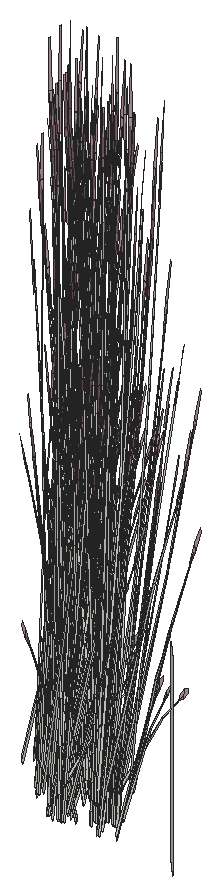
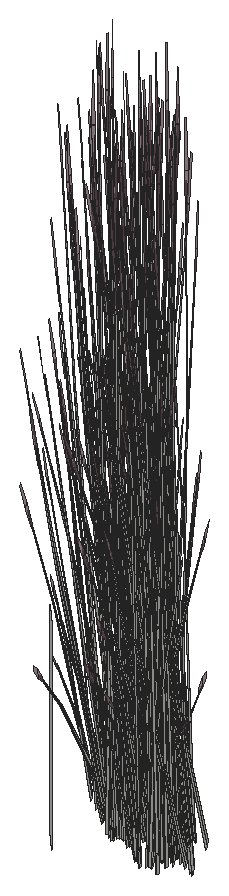
# SketchUp Ruby script. Lengths in inches.
U = 1.inch
M = Sketchup.active_model
def pt(a) = Geom::Point3d.new(a.map { |v| v * U })
def face(e, loops, mat)
  f = e.add_face(loops[0].map { |a| pt(a) })
  loops[1..].each { |l| e.add_face(l.map { |a| pt(a) }).erase! }
  f.material = f.back_material = mat if mat
  f
end
# faces: each face lists its corners as indices into pts; further lists are holes
def faces(e, pts, list, mat = nil) = list.each { |f| face(e, (f[0].is_a?(Array) ? f : [f]).map { |l| l.map { |i| pts[i] } }, mat) }
# xy, xz, yz: faces in a plane at the given z, y or x. An outline is a flat list of corners, or four numbers for a rectangle; further outlines are holes
def ring(l) = l.size == 4 ? [[l[0], l[1]], [l[2], l[1]], [l[2], l[3]], [l[0], l[3]]] : l.each_slice(2).to_a
def flat(e, list, mat, &to3) = list.each { |f| face(e, (f[0].is_a?(Array) ? f : [f]).map { |l| ring(l).map { |u, v| to3.(u, v) } }, mat) }
def xy(e, z, list, mat = nil) = flat(e, list, mat) { |x, y| [x, y, z] }
def xz(e, y, list, mat = nil) = flat(e, list, mat) { |x, z| [x, y, z] }
def yz(e, x, list, mat = nil) = flat(e, list, mat) { |y, z| [x, y, z] }
def lines(e, pts, list) = list.each { |a, b| e.add_line(pt(pts[a]), pt(pts[b])) }
# prism: a flat outline (further loops are holes) pulled along v
def prism(e, loops, v, mat = nil)
  f = face(e, loops, mat); d = Geom::Vector3d.new(v.map { |x| x * U })
  f.pushpull(f.normal.samedirection?(d) ? d.length : -d.length)
end
def box(e, o, s, mat = nil) = prism(e, [[o, [o[0] + s[0], o[1], o[2]], [o[0] + s[0], o[1] + s[1], o[2]], [o[0], o[1] + s[1], o[2]]]], [0, 0, s[2]], mat)
def at(x, y, z, deg = 0) = Geom::Transformation.translation(pt([x, y, z])) * Geom::Transformation.rotation(ORIGIN, Z_AXIS, deg.degrees)
def axes(o, x, y, z) = Geom::Transformation.new([*x, 0, *y, 0, *z, 0, *pt(o).to_a, 1])
def part(name) = M.definitions.add(name)
# library, detail: a bought-in or finely detailed component or shape, given as its bounding box
def library(name, o, s) = part(name).tap { |d| box(d.entities, o, s) }
def detail(e, o, s) = box(e.add_group.entities, o, s)
def put(e, d, t, mat = nil) = e.add_instance(d, t).tap { |i| i.material = mat if mat }
def group(e, t, mat = nil) = e.add_group.tap { |g| g.transformation = t; g.material = mat if mat }.entities
root = M.entities
M.materials.add("LightPink_Translucent").color = [144, 107, 117]
M.materials["LightPink_Translucent"].alpha = 0.75
c1 = part("blade")
p = [[2.15,0.21,22],[0,0.17,0],[0.09,0.45,0],[2.18,0.31,22],[2.29,0.31,22],[0.38,0.45,0],
  [2.48,0.24,33],[2.49,0.24,33],[2.48,0.22,33]]
faces(c1.entities,p,[[0,1,2,3],[4,5,2,3],[6,3,4,7],[8,0,3,6]])
c2 = part("seeds")
p = [[0.3,-0.1,1.38],[-0.01,-0.03,1.59],[-0.01,-0.03,0.03],[0.14,-0.07,-0.07],[0.29,-0.03,3],[0.15,0.01,3.11]]
faces(c2.entities,p,[[0,1,2,3],[1,0,4,5]],"LightPink_Translucent")
c3 = part("blade with seeds")
put(c3.entities,c1,at(0,0,0))
put(c3.entities,c2,axes([2.4,0.25,30.99],[1.5799,-0.05474,1.17369],[-0.12525,1.92788,0.29478],[-0.07173,-0.02425,1.56792]))
p = [[369.42,355.39,618],[371.24,353.33,618],[371.24,353.33,636],[369.42,355.39,636]]
faces(root,p,[[0,1,2,3]])
put(root,c3,axes([359.65,352.5625,623.05],[0.23881,-0.24554,0.35414],[0.22606,0.28036,-0.4572],[-0.0344,0.14245,0.87481]))
put(root,c3,axes([357.41,354.85,622.73],[0.12963,0.31798,0.0643],[-0.23638,0.15564,0.50621],[0.1042,-0.03071,0.77189]))
put(root,c3,axes([361.25,351.21,620.84],[-0.00964,-0.43909,1.41272],[0.43635,0.11382,0.59816],[-0.1032,0.24027,1.3335]))
put(root,c3,axes([356.86,355.74,623.03],[0.0189,-0.47427,-0.1216],[0.35781,0.01296,-0.67495],[0.13781,0.03295,1.02557]))
put(root,c3,axes([357.26,354.86,623.03],[-0.17758,-0.42229,-0.1216],[0.31518,-0.20752,-0.67495],[0.13282,-0.05572,1.02557]))
put(root,c3,axes([362.3,353.98,620.59],[0.12266,0.03828,1.43002],[0.07906,0.39104,-0.30754],[-0.16661,0.0732,0.61141]))
put(root,c3,axes([357.38,354.74,622.73],[-0.09971,0.42522,0.48003],[-0.32782,-0.1454,0.3958],[0.12892,-0.02555,0.9933]))
put(root,c3,axes([359,355.04,620.38],[-0.44609,-0.09826,0.49198],[0.09078,-0.55493,0.19306],[0.06519,0.05359,1.70813]))
put(root,c3,axes([359.61,356.53,620.47],[0.37926,-0.12378,0.17642],[0.09365,0.46065,0.35086],[-0.03382,-0.06712,1.60407]))
put(root,c3,axes([359.5,352.63,623.4],[0.3879,0.02311,-0.13498],[-0.0106,0.43749,-0.74919],[-0.02694,0.1685,1.13838]))
put(root,c3,axes([363.39,352.72,621.34],[0.10032,-0.06746,1.77064],[0.0346,0.47103,0.13857],[-0.2173,0.0625,0.63284]))
put(root,c3,axes([361.01,351.77,620.67],[0.04113,0.53214,-0.29095],[-0.42835,0.03218,-0.50002],[-0.07543,0.07088,1.59708]))
put(root,c3,axes([359.125,355.28,620.21],[0.39487,0,0],[0,0.48281,0],[0,0,1.78407]))
put(root,c3,axes([358.74,354.75,620.72],[-0.21202,-0.39143,0.44739],[0.32115,-0.27564,-0.21531],[0.06861,0.04843,1.43643]))
put(root,c3,axes([358.36,354.84,620.67],[-0.04113,-0.53214,-0.29095],[0.42835,-0.03218,-0.50002],[0.07543,-0.07088,1.59708]))
put(root,c3,axes([360.74,356.55,620.47],[0.10196,-0.46348,0.17642],[0.3731,0.13116,0.35086],[-0.06445,0.00226,1.60407]))
put(root,c3,axes([362.31,353.04,622.72],[-0.05763,0.06055,1.74944],[0.0049,0.44239,-0.27667],[-0.13211,0.05753,0.14031]))
put(root,c3,axes([357.25,354.5,622.68],[0.09562,-0.42421,-0.51099],[0.32782,0.1454,-0.3958],[0.13199,-0.0389,0.97773]))
put(root,c3,axes([360.47,355.59,620.3],[-0.32829,-0.4014,-0.06131],[0.32849,-0.40164,0],[-0.01146,-0.01402,1.75571]))
put(root,c3,axes([358.07,354.77,620.77],[-0.21807,0.07699,1.1486],[0.10265,-0.31819,0.84392],[0.11568,0.02177,0.25299]))
put(root,c3,axes([362.49,352.79,622.53],[-0.29332,-0.1301,-0.35414],[0.08555,-0.37955,0.4572],[-0.11809,0.0348,0.87481]))
put(root,c3,axes([358.3,353.67,620.03],[0.32928,0.11539,-0.30978],[-0.08291,0.40636,0.30978],[0.06638,-0.04686,1.38974]))
put(root,c3,axes([357.45,354.69,622.53],[0.29332,0.1301,-0.35414],[-0.08555,0.37955,0.4572],[0.11809,-0.0348,0.87481]))
put(root,c3,axes([359.81,355.13,620.36],[0.15345,0.52148,0.45755],[-0.43845,0.18134,0.17955],[0.00536,-0.09582,1.58856]))
put(root,c3,axes([359.74,355.07,620.21],[0.17124,-0.42022,-0.44739],[0.35581,0.20224,0.21531],[0,-0.09687,1.43643]))
put(root,c3,axes([360.18,356.42,620.2],[-0.11516,-0.40207,0],[0.32884,-0.1408,0],[0,0,1.54371]))
put(root,c3,axes([361.67,353.49,622.71],[0.04504,0.01251,1.77383],[0.13934,0.41205,-0.16761],[-0.0922,0.10815,0.31391]))
put(root,c3,axes([362.7,352.98,622.68],[-0.09562,0.42421,-0.51099],[-0.32782,-0.1454,-0.3958],[-0.13199,0.0389,0.97773]))
put(root,c3,axes([357.6,354.62,619.98],[-0.22732,0.05597,1.41583],[-0.03618,-0.44548,0.08104],[0.15921,-0.06743,0.80566]))
put(root,c3,axes([358.89,354.64,620.62],[0.06809,-0.4162,0.1448],[0.33266,0.07225,-0.41347],[0.06054,0.04274,1.26744]))
put(root,c3,axes([361.44,353.06,620.375],[0.22066,0.46731,0],[-0.36918,0.26061,-0.51607],[-0.08408,0.05936,1.63711]))
put(root,c3,axes([357.85,354.33,619.49],[-0.01845,-0.0708,1.76342],[0.12793,-0.41416,-0.26939],[0.12905,-0.00596,0.30037]))
put(root,c3,axes([362.53,352.95,619.49],[0.00895,0.0735,1.76342],[-0.18044,0.38382,-0.26939],[-0.12817,-0.01935,0.30037]))
put(root,c3,axes([357.97,356.11,622.71],[-0.03191,-0.04083,1.77383],[0.06981,-0.43764,-0.16761],[0.12571,-0.02796,0.31391]))
put(root,c3,axes([360.32,353.26,623.0625],[-0.34777,-0.12192,0.53283],[0.11892,-0.40083,0.43934],[0.0209,0.15763,1.10256]))
put(root,c3,axes([356.65,354.22,621.875],[-0.14639,0.01056,1.71376],[0.09712,-0.45778,0.13857],[0.20862,0.02831,0.73262]))
put(root,c3,axes([360.22,353.29,622.73],[-0.26007,0.1585,0.0643],[-0.12729,-0.28902,0.50621],[0.02512,0.1274,0.77189]))
put(root,c3,axes([359.36,353.92,620.48],[-0.33032,-0.23318,0.49651],[0.19744,-0.41812,0],[0.07523,0.05311,1.57504]))
put(root,c3,axes([361.09,351.87,620.62],[0.26075,0.2802,0.1448],[-0.2175,0.31612,-0.41347],[-0.06054,0.04274,1.26744]))
put(root,c3,axes([362.05,354.79,620.77],[0.14709,-0.21136,1.1486],[0.05804,0.3346,0.84392],[-0.1063,0.05991,0.25299]))
put(root,c3,axes([359.07,356.35,620.18],[0.37054,-0.15823,-0.19198],[0.1302,0.45581,0.00008],[0.0409,-0.01749,1.73897]))
put(root,c3,axes([357.19,354.65,622.98],[0.31014,-0.20596,-0.71045],[0.17284,0.42397,0.08574],[0.14985,-0.04816,1.00501]))
put(root,c3,axes([360.36,355.18,620.21],[0,-0.53961,0],[0.44133,0,0],[0,0,1.79456]))
put(root,c3,axes([361.17,352.76,620.33],[0.44186,0.15158,0.30756],[-0.11054,0.54181,-0.36492],[-0.07313,0.06781,1.64885]))
put(root,c3,axes([362.68,352.62,623.03],[0.17758,0.42229,-0.1216],[-0.31518,0.20752,-0.67495],[-0.13282,0.05572,1.02557]))
put(root,c3,axes([359.95,355.27,620.43],[0.39767,0.22603,0.24065],[-0.19139,0.46966,0.50002],[0,-0.10827,1.60543]))
put(root,c3,axes([359.82,354.96,620.72],[-0.38326,0.02879,0.44739],[-0.03466,-0.47788,-0.21531],[0.06861,-0.04843,1.43643]))
put(root,c3,axes([362.54,352.625,622.73],[-0.12963,-0.31798,0.0643],[0.23638,-0.15564,0.50621],[-0.1042,0.03071,0.77189]))
put(root,c3,axes([361.36,352.73,620.48],[0.33032,-0.23318,0.49651],[0.19744,0.41812,0],[-0.07523,0.05311,1.57504]))
put(root,c3,axes([362.6,353.88,622.53],[-0.30722,0.06665,-0.35414],[-0.08112,-0.381,0.4572],[-0.08804,0.10234,0.87481]))
put(root,c3,axes([359.64,354.14,620.47],[-0.10196,0.46348,0.17642],[-0.3731,-0.13116,0.35086],[0.06445,-0.00226,1.60407]))
put(root,c3,axes([357.66,355.28,620.59],[-0.085,-0.1147,1.43002],[0.1106,-0.37943,-0.30754],[0.17198,0.0514,0.61141]))
put(root,c3,axes([362.64,353.8,622.73],[-0.08753,-0.42921,0.48003],[0.34336,-0.07449,0.3958],[-0.1012,0.10094,0.9933]))
put(root,c3,axes([360.77,354.16,620.47],[-0.37926,0.12378,0.17642],[-0.09365,-0.46065,0.35086],[0.03382,0.06712,1.60407]))
put(root,c3,axes([361.16,351.56,620.21],[-0.17124,0.42022,-0.44739],[-0.35581,-0.20224,0.21531],[0,0.09687,1.43643]))
put(root,c3,axes([362.57,353.72,622.73],[-0.2423,-0.19613,0.0643],[0.14107,-0.2793,0.50621],[-0.07768,0.0903,0.77189]))
put(root,c3,axes([359.66,354.13,620.03],[0.08291,0.40636,-0.30978],[-0.32928,0.11539,0.30978],[0.06638,0.04686,1.38974]))
put(root,c3,axes([360.15,354.84,620.36],[-0.29264,0.42323,0.45755],[-0.34767,-0.3736,0.17955],[0.07055,-0.04224,1.58856]))
put(root,c3,axes([358.85,354.78,620.67],[0.35635,-0.30962,-0.29095],[0.23697,0.43749,-0.50002],[0.08792,0.04443,1.59708]))
put(root,c3,axes([359.91,354.72,623.05],[-0.30722,0.06665,0.35414],[-0.08112,-0.381,-0.4572],[0.08804,-0.10234,0.87481]))
put(root,c3,axes([360.32,352.96,623.05],[0.1064,-0.35863,0.35414],[0.31043,0.1046,-0.4572],[0.02846,0.14439,0.87481]))
put(root,c3,axes([362.8,352.74,623.05],[0.29332,0.1301,0.35414],[-0.08555,0.37955,-0.4572],[-0.11809,0.0348,0.87481]))
put(root,c3,axes([360.53,355.05,620.38],[-0.44609,-0.09826,0.49198],[0.09078,-0.55493,0.19306],[0.06519,0.05359,1.70813]))
put(root,c3,axes([360.89,352.37,620.29],[0.15345,0.53576,-0.06012],[-0.43845,0.18773,0],[0.00536,0.01871,1.72173]))
put(root,c3,axes([360.66,355.3,620.21],[0.39487,0,0],[0,0.48281,0],[0,0,1.78407]))
put(root,c3,axes([362.16,351.66,620.2],[-0.44111,-0.00373,-0.04976],[0,-0.52122,0.49943],[-0.01386,0.11865,1.58352]))
put(root,c3,axes([360.28,354.76,620.72],[-0.21202,-0.39143,0.44739],[0.32115,-0.27564,-0.21531],[0.06861,0.04843,1.43643]))
put(root,c3,axes([359.89,354.86,620.67],[-0.04113,-0.53214,-0.29095],[0.42835,-0.03218,-0.50002],[0.07543,-0.07088,1.59708]))
put(root,c3,axes([357.95,354.5,619.59],[-0.3474,0.18671,1.28929],[-0.11057,-0.53572,0.50096],[0.21332,0.00891,1.46642]))
put(root,c3,axes([360.74,354.24,623.65],[0.2439,-0.26754,-0.06488],[0.22348,0.29302,-0.29416],[0.01573,0.08303,0.97024]))
put(root,c3,axes([363.23,354.51,620.02],[-0.33032,-0.23318,-0.49651],[0.19744,-0.41812,0],[-0.07523,-0.05311,1.57504]))
put(root,c3,axes([359.55,353.67,620.375],[0.22066,-0.46731,0],[0.36918,0.26061,-0.51607],[0.08408,0.05936,1.63711]))
put(root,c3,axes([359.84,353.68,620.03],[0.32928,0.11539,-0.30978],[-0.08291,0.40636,0.30978],[0.06638,-0.04686,1.38974]))
put(root,c3,axes([361.02,352.54,620.2],[0.35581,0.20937,0],[-0.17124,0.43505,0],[0,0,1.74954]))
put(root,c3,axes([363.43,354.79,620.375],[-0.22066,0.46731,0],[-0.36918,-0.26061,-0.51607],[-0.08408,-0.05936,1.63711]))
put(root,c3,axes([359.75,353.95,620.02],[0.33032,0.23318,-0.49651],[-0.19744,0.41812,0],[0.07523,0.05311,1.57504]))
put(root,c3,axes([360.22,353.12,623.03],[0.34538,-0.21713,-0.1216],[0.16972,0.38536,-0.67495],[0.04557,0.16239,1.02557]))
put(root,c3,axes([362.07,351.74,620.03],[-0.24637,0.29097,-0.30978],[-0.24637,-0.29097,0.30978],[0,0.09372,1.38974]))
put(root,c3,axes([360.42,354.65,620.62],[0.06809,-0.4162,0.1448],[0.33266,0.07225,-0.41347],[0.06054,0.04274,1.26744]))
put(root,c3,axes([359.96,355.63,623.05],[-0.29332,-0.1301,0.35414],[0.08555,-0.37955,-0.4572],[0.11809,-0.0348,0.87481]))
put(root,c3,axes([362.85,353.65,623.05],[0.30722,-0.06665,0.35414],[0.08112,0.381,-0.4572],[-0.08804,0.10234,0.87481]))
put(root,c3,axes([361.36,351.6875,620.09],[0.12941,0.42699,-0.69212],[-0.37279,0.15378,-0.18165],[0.0143,0.14459,1.52773]))
put(root,c3,axes([360.83,355.125,620.26],[-0.21881,-0.29821,-0.06488],[0.23965,-0.27324,-0.29416],[0.0679,-0.01924,0.97024]))
put(root,c3,axes([360.9,353.93,620.48],[-0.33032,-0.23318,0.49651],[0.19744,-0.41812,0],[0.07523,0.05311,1.57504]))
put(root,c3,axes([360.61,356.36,620.18],[0.37054,-0.15823,-0.19198],[0.1302,0.45581,0.00008],[0.0409,-0.01749,1.73897]))
put(root,c3,axes([360.1875,354.66,622.73],[0.2423,0.19613,0.0643],[-0.14107,0.2793,0.50621],[0.07768,-0.0903,0.77189]))
put(root,c3,axes([361.21,351.21,620.67],[0.39748,0.22252,-0.29095],[-0.19139,0.46966,-0.50002],[0.01249,0.11531,1.59708]))
put(root,c3,axes([364.13,353.6875,620.67],[-0.35635,0.30962,-0.29095],[-0.23697,-0.43749,-0.50002],[-0.08792,-0.04443,1.59708]))
put(root,c3,axes([360.12,354.58,622.73],[0.08753,0.42921,0.48003],[-0.34336,0.07449,0.3958],[0.1012,-0.10094,0.9933]))
put(root,c3,axes([363.32,354.34,620.03],[-0.08291,-0.40636,-0.30978],[0.32928,-0.11539,0.30978],[-0.06638,-0.04686,1.38974]))
put(root,c3,axes([362.24,351.75,620.02],[0,0.46636,-0.49651],[-0.39487,0,0],[0,0.10622,1.57504]))
put(root,c3,axes([361.18,353.16,622.73],[-0.35104,0.10702,0.48003],[-0.06092,-0.41983,0.3958],[0.08256,0.12373,0.9933]))
put(root,c3,axes([361.12,353.25,622.73],[-0.16041,0.29625,0.0643],[-0.22843,-0.17248,0.50621],[0.07385,0.09498,0.77189]))
put(root,c3,axes([360.23,355.75,622.73],[0.12963,0.31798,0.0643],[-0.23638,0.15564,0.50621],[0.1042,-0.03071,0.77189]))
put(root,c3,axes([360.08,355.76,623.03],[-0.17758,-0.42229,-0.1216],[0.31518,-0.20752,-0.67495],[0.13282,-0.05572,1.02557]))
put(root,c3,axes([360.2,355.64,622.73],[-0.09971,0.42522,0.48003],[-0.32782,-0.1454,0.3958],[0.12892,-0.02555,0.9933]))
put(root,c3,axes([364.53,353.83,620.46],[-0.34464,-0.37536,-0.25192],[0.29,-0.42149,0.5513],[-0.0928,0.04391,1.68216]))
put(root,c3,axes([361.19,354.14,620.03],[0.08291,0.40636,-0.30978],[-0.32928,0.11539,0.30978],[0.06638,0.04686,1.38974]))
put(root,c3,axes([360.39,354.79,620.67],[0.35635,-0.30962,-0.29095],[0.23697,0.43749,-0.50002],[0.08792,0.04443,1.59708]))
put(root,c3,axes([364.35,353.75,620.21],[-0.38326,0.02879,-0.44739],[-0.03466,-0.47788,0.21531],[-0.06861,0.04843,1.43643]))
put(root,c3,axes([361.07,352.9,623.05],[-0.05451,-0.37564,0.35414],[0.31161,-0.09919,-0.4572],[0.0837,0.10765,0.87481]))
put(root,c3,axes([361.45,354.74,623.05],[-0.30722,0.06665,0.35414],[-0.08112,-0.381,-0.4572],[0.08804,-0.10234,0.87481]))
put(root,c3,axes([360.07,355.4,622.68],[0.09562,-0.42421,-0.51099],[0.32782,0.1454,-0.3958],[0.13199,-0.0389,0.97773]))
put(root,c3,axes([361.28,350.74,622.47],[-0.30498,-0.24231,1.38283],[0.32203,-0.37727,0.59665],[0.0984,0.22736,1.33663]))
put(root,c3,axes([363.62,354.55,620.48],[0.33032,0.23318,0.49651],[-0.19744,0.41812,0],[-0.07523,-0.05311,1.57504]))
put(root,c3,axes([360.76,353.43,622.71],[0.00104,-0.05646,1.77383],[0.30246,-0.2491,-0.16761],[0.10506,0.08891,0.31391]))
put(root,c3,axes([361.74,352.72,620.77],[-0.19872,-0.13409,1.1486],[0.2566,-0.13625,0.84392],[0.06921,0.11541,0.25299]))
put(root,c3,axes([361.03,352.57,620.59],[0.00623,-0.15459,1.43002],[0.29764,-0.17268,-0.30754],[0.09188,0.18503,0.61141]))
put(root,c3,axes([360.27,355.59,622.53],[0.29332,0.1301,-0.35414],[-0.08555,0.37955,0.4572],[0.11809,-0.0348,0.87481]))
put(root,c3,axes([359.49,354.51,619.59],[-0.3474,0.18671,1.28929],[-0.11057,-0.53572,0.50096],[0.21332,0.00891,1.46642]))
put(root,c3,axes([364.09,353.82,620.62],[-0.06809,0.4162,0.1448],[-0.33266,-0.07225,-0.41347],[-0.06054,-0.04274,1.26744]))
put(root,c3,axes([364.78,354.86,620.19],[-0.21791,-0.46895,-0.05142],[0.36918,-0.26061,0.51607],[-0.09097,0.04465,1.6363]))
put(root,c3,axes([360.42,355.52,619.98],[-0.22732,0.05597,1.41583],[-0.03618,-0.44548,0.08104],[0.15921,-0.06743,0.80566]))
put(root,c3,axes([362.34,351.4,620.375],[0.44133,0,0],[0,0.52122,-0.51607],[0,0.11871,1.63711]))
put(root,c3,axes([360.67,355.23,619.49],[-0.01845,-0.0708,1.76342],[0.12793,-0.41416,-0.26939],[0.12905,-0.00596,0.30037]))
put(root,c3,axes([361.09,353.68,620.375],[0.22066,-0.46731,0],[0.36918,0.26061,-0.51607],[0.08408,0.05936,1.63711]))
put(root,c3,axes([364.68,354.8,620.03],[-0.32928,-0.11539,-0.30978],[0.08291,-0.40636,0.30978],[-0.06638,0.04686,1.38974]))
put(root,c3,axes([359.47,355.125,621.875],[-0.14639,0.01056,1.71376],[0.09712,-0.45778,0.13857],[0.20862,0.02831,0.73262]))
put(root,c3,axes([361.29,353.97,620.02],[0.33032,0.23318,-0.49651],[-0.19744,0.41812,0],[0.07523,0.05311,1.57504]))
put(root,c3,axes([361.77,353.33,620.67],[-0.22633,-0.01463,1.0506],[0.14947,-0.31064,0.58006],[0.08941,0.11036,0.8241]))
put(root,c3,axes([360.01,355.55,622.98],[0.31014,-0.20596,-0.71045],[0.17284,0.42397,0.08574],[0.14985,-0.04816,1.00501]))
put(root,c3,axes([364.62,353.62,620.67],[0.04113,0.53214,-0.29095],[-0.42835,0.03218,-0.50002],[-0.07543,0.07088,1.59708]))
put(root,c3,axes([361.5,355.65,623.05],[-0.29332,-0.1301,0.35414],[0.08555,-0.37955,-0.4572],[0.11809,-0.0348,0.87481]))
put(root,c3,axes([361.04,353.1,623.03],[0.21031,-0.39918,-0.1216],[0.30457,0.22997,-0.67495],[0.10587,0.11278,1.02557]))
put(root,c3,axes([361.05,355.1,622.72],[0.04898,-0.07104,1.74944],[-0.06269,-0.43574,-0.27667],[0.12289,-0.08262,0.14031]))
put(root,c3,axes([362.37,355.14,620.26],[-0.21881,-0.29821,-0.06488],[0.23965,-0.27324,-0.29416],[0.0679,-0.01924,0.97024]))
put(root,c3,axes([363.98,353.43,620.36],[0.44609,0.09826,0.45755],[-0.09078,0.55493,0.17955],[-0.06519,-0.05359,1.58856]))
put(root,c3,axes([361.73,354.68,622.73],[0.2423,0.19613,0.0643],[-0.14107,0.2793,0.50621],[0.07768,-0.0903,0.77189]))
put(root,c3,axes([361.29,352.9,622.68],[0.34827,-0.11086,-0.51099],[0.06092,0.41983,-0.3958],[0.09354,0.12031,0.97773]))
put(root,c3,axes([361.66,354.59,622.73],[0.08753,0.42921,0.48003],[-0.34336,0.07449,0.3958],[0.1012,-0.10094,0.9933]))
put(root,c3,axes([361.6875,352.4,623.05],[-0.20082,-0.29199,0.35414],[0.2293,-0.2764,-0.4572],[0.1165,0.04206,0.87481]))
put(root,c3,axes([361.87,352.66,622.73],[-0.01777,0.35463,0.0643],[-0.26836,-0.00972,0.50621],[0.1028,0.03711,0.77189]))
put(root,c3,axes([361.79,353.22,619.49],[0.02571,-0.06733,1.76342],[0.32373,-0.19829,-0.26939],[0.09815,0.10263,0.30037]))
put(root,c3,axes([361.89,352.55,622.73],[-0.26024,0.30729,0.48003],[-0.22444,-0.32634,0.3958],[0.1221,0.05668,0.9933]))
put(root,c3,axes([363.74,354.3125,620.47],[0.37926,-0.12378,0.17642],[0.09365,0.46065,0.35086],[-0.03382,-0.06712,1.60407]))
put(root,c3,axes([364.23,354.39,620.2],[-0.35581,-0.20937,0],[0.17124,-0.43505,0],[0,0,1.62707]))
put(root,c3,axes([361.76,355.77,622.73],[0.12963,0.31798,0.0643],[-0.23638,0.15564,0.50621],[0.1042,-0.03071,0.77189]))
put(root,c3,axes([361.62,355.77,623.03],[-0.17758,-0.42229,-0.1216],[0.31518,-0.20752,-0.67495],[0.13282,-0.05572,1.02557]))
put(root,c3,axes([361.74,355.65,622.73],[-0.09971,0.42522,0.48003],[-0.32782,-0.1454,0.3958],[0.12892,-0.02555,0.9933]))
put(root,c3,axes([364.87,354.34,620.47],[0.10196,-0.46348,0.17642],[0.3731,0.13116,0.35086],[-0.06445,0.00226,1.60407]))
put(root,c3,axes([364.7,353.72,620.62],[0.26075,0.2802,0.1448],[-0.2175,0.31612,-0.41347],[-0.06054,0.04274,1.26744]))
put(root,c3,axes([364.69,353.52,620.72],[0.38326,-0.02879,0.44739],[0.03466,0.47788,-0.21531],[-0.06861,0.04843,1.43643]))
put(root,c3,axes([364.98,354.59,620.48],[0.33032,-0.23318,0.49651],[0.19744,0.41812,0],[-0.07523,0.05311,1.57504]))
put(root,c3,axes([361.25,351.8,621.875],[-0.1311,-0.08035,1.71376],[0.27131,-0.33708,0.13857],[0.16909,0.15206,0.73262]))
put(root,c3,axes([361.6,355.41,622.68],[0.09562,-0.42421,-0.51099],[0.32782,0.1454,-0.3958],[0.13199,-0.0389,0.97773]))
put(root,c3,axes([364.3125,354.21,620.2],[-0.11516,-0.40207,0],[0.32884,-0.1408,0],[0,0,1.54371]))
put(root,c3,axes([361.97,352.55,622.53],[0.20082,0.29199,-0.35414],[-0.2293,0.2764,0.4572],[0.1165,0.04206,0.87481]))
put(root,c3,axes([361.8,355.61,622.53],[0.29332,0.1301,-0.35414],[-0.08555,0.37955,0.4572],[0.11809,-0.0348,0.87481]))
put(root,c3,axes([364.78,353.41,620.21],[-0.17124,0.42022,-0.44739],[-0.35581,-0.20224,0.21531],[0,0.09687,1.43643]))
put(root,c3,axes([361.95,355.53,619.98],[-0.22732,0.05597,1.41583],[-0.03618,-0.44548,0.08104],[0.15921,-0.06743,0.80566]))
put(root,c3,axes([362.2,355.24,619.49],[-0.01845,-0.0708,1.76342],[0.12793,-0.41416,-0.26939],[0.12905,-0.00596,0.30037]))
put(root,c3,axes([365.45,353.16,620.47],[-0.2773,-0.3397,0.17642],[0.27945,-0.32949,0.35086],[-0.03063,0.06937,1.60407]))
put(root,c3,axes([361.01,355.14,621.875],[-0.14639,0.01056,1.71376],[0.09712,-0.45778,0.13857],[0.20862,0.02831,0.73262]))
put(root,c3,axes([364.72,353.18,620.29],[0,0.53934,-0.05637],[-0.44133,0,0],[0,0.01695,1.79368]))
put(root,c3,axes([362.05,352.3,622.72],[0.07571,-0.00789,1.74944],[0.20767,-0.36231,-0.27667],[0.13467,0.04783,0.14031]))
put(root,c3,axes([364.51,354.22,620.29],[0.15345,0.53576,-0.06012],[-0.43845,0.18773,0],[0.00536,0.01871,1.72173]))
put(root,c3,axes([361.54,355.57,622.98],[0.31014,-0.20596,-0.71045],[0.17284,0.42397,0.08574],[0.14985,-0.04816,1.00501]))
put(root,c3,axes([362.58,355.11,622.72],[0.04898,-0.07104,1.74944],[-0.06269,-0.43574,-0.27667],[0.12289,-0.08262,0.14031]))
put(root,c3,axes([365.78,353.52,620.2],[-0.44111,-0.00373,-0.04976],[0,-0.52122,0.49943],[-0.01386,0.11865,1.58352]))
put(root,c3,axes([364.91,351.95,620.47],[-0.37926,0.12378,0.17642],[-0.09365,-0.46065,0.35086],[0.03382,0.06712,1.60407]))
put(root,c3,axes([361.76,352.36,622.98],[0.35281,0.01123,-0.71045],[-0.0237,0.47284,0.08574],[0.14947,0.0499,1.00501]))
put(root,c3,axes([364.79,353.29,620.21],[0.24637,0.30123,0],[-0.24637,0.30123,0],[0,0,1.69266]))
put(root,c3,axes([364.78,352.9375,620.72],[0.17124,-0.42022,0.44739],[0.35581,0.20224,-0.21531],[0,0.09687,1.43643]))
put(root,c3,axes([364.64,354.4,620.2],[0.35581,0.20937,0],[-0.17124,0.43505,0],[0,0,1.74954]))
put(root,c3,axes([364.67,352.84,620.38],[-0.44609,-0.09826,0.49198],[0.09078,-0.55493,0.19306],[0.06519,0.05359,1.70813]))
put(root,c3,axes([365.68,353.59,620.03],[-0.24637,0.29097,-0.30978],[-0.24637,-0.29097,0.30978],[0,0.09372,1.38974]))
put(root,c3,axes([364.8,353.08,620.21],[0.39487,0,0],[0,0.48281,0],[0,0,1.78407]))
put(root,c3,axes([364.42,352.55,620.72],[-0.21202,-0.39143,0.44739],[0.32115,-0.27564,-0.21531],[0.06861,0.04843,1.43643]))
put(root,c3,axes([364.93,353.03,620.62],[0.32884,-0.136,0.1448],[0.11516,0.38837,-0.41347],[0,0.08547,1.26744]))
put(root,c3,axes([362.54,352.125,620.59],[-0.085,-0.1147,1.43002],[0.1106,-0.37943,-0.30754],[0.17198,0.0514,0.61141]))
put(root,c3,axes([364.82,353.0625,620.67],[0.39748,0.22252,-0.29095],[-0.19139,0.46966,-0.50002],[0.01249,0.11531,1.59708]))
put(root,c3,axes([365.68,353.17,620.48],[0,-0.46636,0.49651],[0.39487,0,0],[0,0.10622,1.57504]))
put(root,c3,axes([364.74,354.15,620.18],[0.37054,-0.15823,-0.19198],[0.1302,0.45581,0.00008],[0.0409,-0.01749,1.73897]))
put(root,c3,axes([364.75,352.79,620.21],[0.21202,0.39143,-0.44739],[-0.32115,0.27564,0.21531],[0.06861,0.04843,1.43643]))
put(root,c3,axes([365.33,351.93,620.03],[0.08291,0.40636,-0.30978],[-0.32928,0.11539,0.30978],[0.06638,0.04686,1.38974]))
put(root,c3,axes([365.95,353.25,620.375],[0.44133,0,0],[0,0.52122,-0.51607],[0,0.11871,1.63711]))
put(root,c3,axes([364.53,352.57,620.67],[0.35635,-0.30962,-0.29095],[0.23697,0.43749,-0.50002],[0.08792,0.04443,1.59708]))
put(root,c3,axes([365.3,354.25,623.05],[-0.20082,-0.29199,0.35414],[0.2293,-0.2764,-0.4572],[0.1165,0.04206,0.87481]))
put(root,c3,axes([365.42,351.75,620.02],[0.33032,0.23318,-0.49651],[-0.19744,0.41812,0],[0.07523,0.05311,1.57504]))
put(root,c3,axes([365.48,354.52,622.73],[-0.01777,0.35463,0.0643],[-0.26836,-0.00972,0.50621],[0.1028,0.03711,0.77189]))
put(root,c3,axes([365.51,354.4,622.73],[-0.26024,0.30729,0.48003],[-0.22444,-0.32634,0.3958],[0.1221,0.05668,0.9933]))
put(root,c3,axes([366.19,354.45,621.93],[-0.06755,-0.39203,-0.03492],[0.31928,-0.09013,-0.15832],[0.06667,0.02485,0.52218]))
put(root,c3,axes([364.94,352.64,620.06],[0.36714,0.07646,-0.62353],[-0.07747,0.47163,-0.16365],[0.10956,0.05715,1.37633]))
put(root,c3,axes([365.9,353.55,622.73],[0.12963,0.31798,0.0643],[-0.23638,0.15564,0.50621],[0.1042,-0.03071,0.77189]))
put(root,c3,axes([365.59,354.4,622.53],[0.20082,0.29199,-0.35414],[-0.2293,0.2764,0.4572],[0.1165,0.04206,0.87481]))
put(root,c3,axes([365.36,354.4375,623.03],[0.0189,-0.47427,-0.1216],[0.35781,0.01296,-0.67495],[0.13781,0.03295,1.02557]))
put(root,c3,axes([365.875,353.4375,622.73],[-0.09971,0.42522,0.48003],[-0.32782,-0.1454,0.3958],[0.12892,-0.02555,0.9933]))
put(root,c3,axes([365.67,354.15,622.72],[0.07571,-0.00789,1.74944],[0.20767,-0.36231,-0.27667],[0.13467,0.04783,0.14031]))
put(root,c3,axes([366.5625,353.47,620.77],[-0.21807,0.07699,1.1486],[0.10265,-0.31819,0.84392],[0.11568,0.02177,0.25299]))
put(root,c3,axes([365.94,353.39,622.53],[0.29332,0.1301,-0.35414],[-0.08555,0.37955,0.4572],[0.11809,-0.0348,0.87481]))
put(root,c3,axes([365.375,354.21,622.98],[0.35281,0.01123,-0.71045],[-0.0237,0.47284,0.08574],[0.14947,0.0499,1.00501]))
put(root,c3,axes([366.34,353.03,619.49],[-0.01845,-0.0708,1.76342],[0.12793,-0.41416,-0.26939],[0.12905,-0.00596,0.30037]))
put(root,c3,axes([366.46,354.8125,622.71],[-0.03191,-0.04083,1.77383],[0.06981,-0.43764,-0.16761],[0.12571,-0.02796,0.31391]))
put(root,c3,axes([365.14,352.92,621.875],[-0.14639,0.01056,1.71376],[0.09712,-0.45778,0.13857],[0.20862,0.02831,0.73262]))
put(root,c3,axes([366.16,353.98,620.59],[-0.085,-0.1147,1.43002],[0.1106,-0.37943,-0.30754],[0.17198,0.0514,0.61141]))
